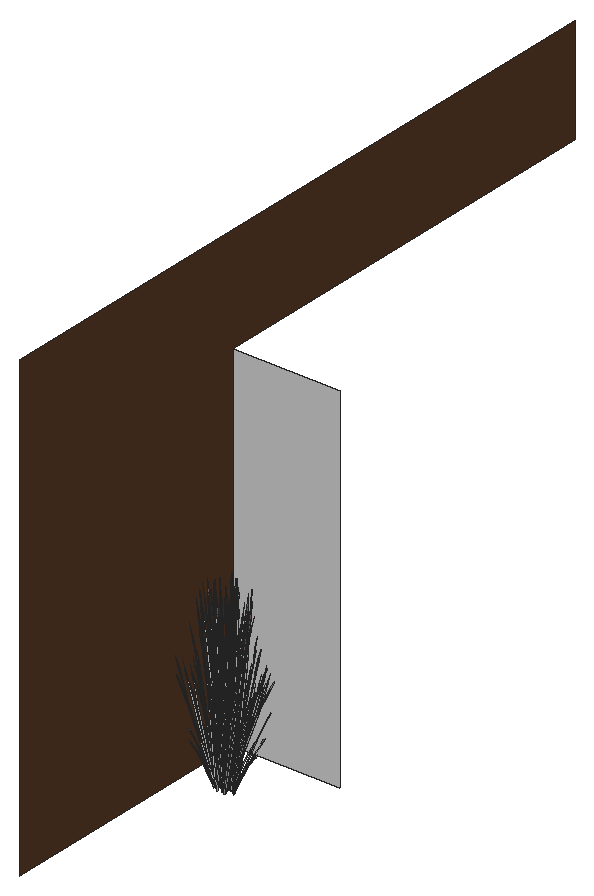
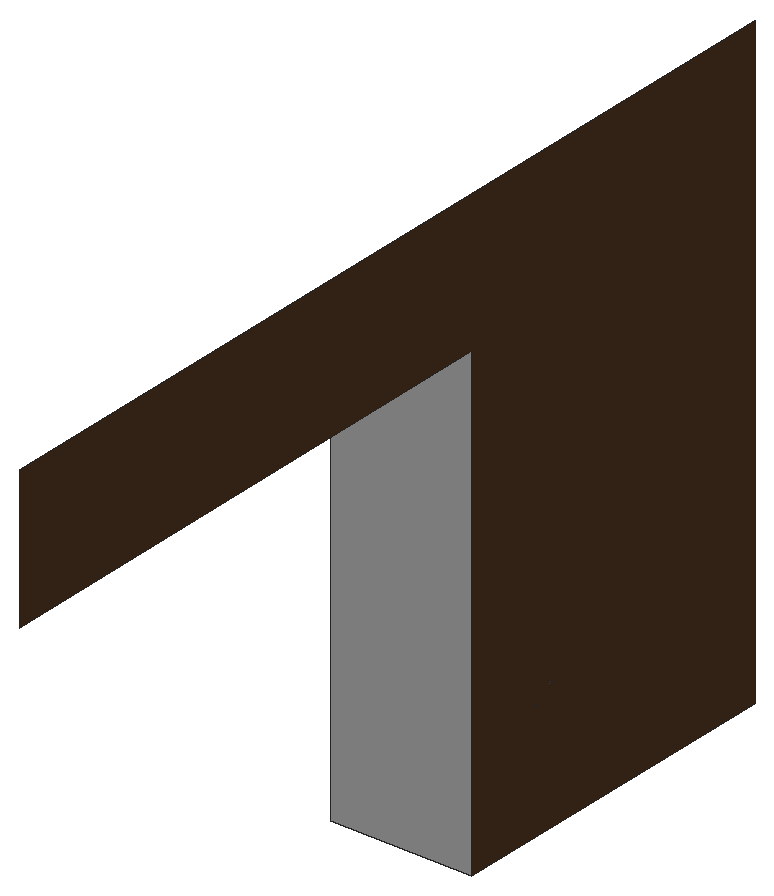
# SketchUp Ruby script. Lengths in inches.
U = 1.inch
M = Sketchup.active_model
def pt(a) = Geom::Point3d.new(a.map { |v| v * U })
def face(e, loops, mat)
  f = e.add_face(loops[0].map { |a| pt(a) })
  loops[1..].each { |l| e.add_face(l.map { |a| pt(a) }).erase! }
  f.material = f.back_material = mat if mat
  f
end
# faces: each face lists its corners as indices into pts; further lists are holes
def faces(e, pts, list, mat = nil) = list.each { |f| face(e, (f[0].is_a?(Array) ? f : [f]).map { |l| l.map { |i| pts[i] } }, mat) }
# xy, xz, yz: faces in a plane at the given z, y or x. An outline is a flat list of corners, or four numbers for a rectangle; further outlines are holes
def ring(l) = l.size == 4 ? [[l[0], l[1]], [l[2], l[1]], [l[2], l[3]], [l[0], l[3]]] : l.each_slice(2).to_a
def flat(e, list, mat, &to3) = list.each { |f| face(e, (f[0].is_a?(Array) ? f : [f]).map { |l| ring(l).map { |u, v| to3.(u, v) } }, mat) }
def xy(e, z, list, mat = nil) = flat(e, list, mat) { |x, y| [x, y, z] }
def xz(e, y, list, mat = nil) = flat(e, list, mat) { |x, z| [x, y, z] }
def yz(e, x, list, mat = nil) = flat(e, list, mat) { |y, z| [x, y, z] }
def lines(e, pts, list) = list.each { |a, b| e.add_line(pt(pts[a]), pt(pts[b])) }
# prism: a flat outline (further loops are holes) pulled along v
def prism(e, loops, v, mat = nil)
  f = face(e, loops, mat); d = Geom::Vector3d.new(v.map { |x| x * U })
  f.pushpull(f.normal.samedirection?(d) ? d.length : -d.length)
end
def box(e, o, s, mat = nil) = prism(e, [[o, [o[0] + s[0], o[1], o[2]], [o[0] + s[0], o[1] + s[1], o[2]], [o[0], o[1] + s[1], o[2]]]], [0, 0, s[2]], mat)
def at(x, y, z, deg = 0) = Geom::Transformation.translation(pt([x, y, z])) * Geom::Transformation.rotation(ORIGIN, Z_AXIS, deg.degrees)
def axes(o, x, y, z) = Geom::Transformation.new([*x, 0, *y, 0, *z, 0, *pt(o).to_a, 1])
def part(name) = M.definitions.add(name)
# library, detail: a bought-in or finely detailed component or shape, given as its bounding box
def library(name, o, s) = part(name).tap { |d| box(d.entities, o, s) }
def detail(e, o, s) = box(e.add_group.entities, o, s)
def put(e, d, t, mat = nil) = e.add_instance(d, t).tap { |i| i.material = mat if mat }
def group(e, t, mat = nil) = e.add_group.tap { |g| g.transformation = t; g.material = mat if mat }.entities
root = M.entities
M.materials.add("LightPink_Translucent").color = [144, 107, 117]
M.materials["LightPink_Translucent"].alpha = 0.75
M.materials.add("Wood_Veneer_15_1K").color = [81, 54, 35]
M.materials.add("[_0053_Ivory_]").color = [200, 200, 200]
c1 = part("blade")
p = [[2.15,0.21,22],[0,0.17,0],[0.09,0.45,0],[2.18,0.31,22],[2.29,0.31,22],[0.38,0.45,0],
  [2.48,0.24,33],[2.49,0.24,33],[2.48,0.22,33]]
faces(c1.entities,p,[[0,1,2,3],[4,5,2,3],[6,3,4,7],[8,0,3,6]])
c2 = part("seeds")
p = [[0.3,-0.1,1.38],[-0.01,-0.03,1.59],[-0.01,-0.03,0.03],[0.14,-0.07,-0.07],[0.29,-0.03,3],[0.15,0.01,3.11]]
faces(c2.entities,p,[[0,1,2,3],[1,0,4,5]],"LightPink_Translucent")
c3 = part("blade with seeds")
put(c3.entities,c1,at(0,0,0))
put(c3.entities,c2,axes([2.4,0.25,30.99],[1.5799,-0.05474,1.17369],[-0.12525,1.92788,0.29478],[-0.07173,-0.02425,1.56792]))
xz(root,359.15,[[617.51,252,653.51,372]],"[_0053_Ivory_]")
yz(root,617.51,[[269.15,252,359.15,252,359.15,372,503.15,372,503.15,408,269.15,408]],"Wood_Veneer_15_1K")
put(root,c3,axes([631.41,334.82,253.68],[0.56663,0.1556,-0.30978],[-0.14267,0.54795,0.30978],[0.11423,-0.06319,1.38974]),"[_0053_Ivory_]")
put(root,c3,axes([629.83,335.5,256.63],[-0.60713,-0.01514,-0.71045],[0.04078,-0.63759,0.08574],[-0.25721,-0.06729,1.00501]),"[_0053_Ivory_]")
put(root,c3,axes([629.8,336.73,253.98],[-0.56493,0.5287,0.30756],[-0.56528,-0.52313,-0.36492],[-0.01973,-0.15014,1.64885]),"[_0053_Ivory_]")
put(root,c3,axes([631.6,336.97,254.09],[0.68433,0.30479,0.24065],[-0.32934,0.63331,0.50002],[0,-0.14599,1.60543]),"[_0053_Ivory_]")
put(root,c3,axes([631.33,337.83,254.09],[0.16098,-0.74515,-0.23429],[0.76326,0.12989,0.51271],[-0.13337,-0.1029,1.5644]),"[_0053_Ivory_]")
put(root,c3,axes([629.63,335.63,256.33],[-0.44101,0.41656,-0.51099],[-0.38623,-0.44004,-0.3958],[-0.22407,-0.06338,0.97773]),"[_0053_Ivory_]")
put(root,c3,axes([628.64,336.18,254.42],[0.38775,-0.045,1.1486],[-0.24596,0.39648,0.84392],[-0.19161,-0.05948,0.25299]),"[_0053_Ivory_]")
put(root,c3,axes([631.38,336.55,254.37],[-0.65953,0.03882,0.44739],[-0.05964,-0.64439,-0.21531],[0.11807,-0.06531,1.43643]),"[_0053_Ivory_]")
put(root,c3,axes([629.68,337.02,254.13],[0,0.62885,0.49651],[-0.67951,0,0],[0,-0.14322,1.57504]),"[_0053_Ivory_]")
put(root,c3,axes([634.45,337.16,256.33],[0.16454,-0.57202,-0.51099],[0.56413,0.19607,-0.3958],[0.22713,-0.05245,0.97773]),"[_0053_Ivory_]")
put(root,c3,axes([633.55,334.83,254.03],[0.37973,-0.63014,0],[0.6353,0.35142,-0.51607],[0.14469,0.08004,1.63711]),"[_0053_Ivory_]")
put(root,c3,axes([629.08,336.07,255.53],[0.25192,-0.01424,1.71376],[-0.16712,0.61729,0.13857],[-0.35901,-0.03818,0.73262]),"[_0053_Ivory_]")
put(root,c3,axes([631.28,337.53,253.86],[-0.36485,-0.52782,-0.44739],[0.55265,-0.37168,0.21531],[-0.11807,-0.06531,1.43643]),"[_0053_Ivory_]")
put(root,c3,axes([631.36,336.78,254.01],[0.26406,0.70318,0.45755],[-0.7545,0.24452,0.17955],[0.00922,-0.12921,1.58856]),"[_0053_Ivory_]")
put(root,c3,axes([635.05,337.32,253.64],[-0.39118,0.07547,1.41583],[-0.06226,-0.6007,0.08104],[0.27398,-0.09092,0.80566]),"[_0053_Ivory_]")
put(root,c3,axes([635.76,336.79,253.91],[-0.37654,-0.40212,-0.06488],[0.4124,-0.36845,-0.29416],[0.11685,-0.02594,0.97024]),"[_0053_Ivory_]")
put(root,c3,axes([631.22,337.33,254.37],[-0.29468,0.56664,0.44739],[-0.61229,-0.27271,-0.21531],[0,-0.13062,1.43643]),"[_0053_Ivory_]")
put(root,c3,axes([632.31,336.84,253.86],[0,-0.72763,0],[0.75945,0,0],[0,0,1.79456]),"[_0053_Ivory_]")
put(root,c3,axes([633.23,335.16,254.13],[-0.56842,-0.31443,0.49651],[0.33976,-0.56381,0],[0.12946,0.07161,1.57504]),"[_0053_Ivory_]")
put(root,c3,axes([634.34,337.37,256.63],[0.53369,-0.27773,-0.71045],[0.29743,0.5717,0.08574],[0.25786,-0.06494,1.00501]),"[_0053_Ivory_]")
put(root,c3,axes([630.95,337.73,253.71],[-0.63179,-0.1031,-0.62353],[0.13332,-0.63596,-0.16365],[-0.18854,-0.07706,1.37633]),"[_0053_Ivory_]")
put(root,c3,axes([631.95,336.38,254.01],[-0.50358,0.57069,0.45755],[-0.59827,-0.50377,0.17955],[0.1214,-0.05695,1.58856]),"[_0053_Ivory_]")
put(root,c3,axes([632.5,337.4,253.95],[-0.56493,-0.54126,-0.06131],[0.56528,-0.54159,0],[-0.01973,-0.0189,1.75571]),"[_0053_Ivory_]")
put(root,c3,axes([631.07,335.44,254.13],[-0.17545,0.62497,0.17642],[-0.64204,-0.17686,0.35086],[0.11091,-0.00304,1.60407]),"[_0053_Ivory_]")
put(root,c3,axes([630.81,335.95,253.25],[-0.59782,0.25177,1.28929],[-0.19028,-0.72239,0.50096],[0.36709,0.01202,1.46642]),"[_0053_Ivory_]")
put(root,c3,axes([632.41,336.14,254.27],[0.11717,-0.56122,0.1448],[0.57245,0.09742,-0.41347],[0.10418,0.05763,1.26744]),"[_0053_Ivory_]")
put(root,c3,axes([631.42,337.47,254.01],[0.76764,0.13249,0.45755],[-0.15622,0.74829,0.17955],[-0.11218,-0.07226,1.58856]),"[_0053_Ivory_]")
put(root,c3,axes([635.48,336.93,253.15],[-0.03174,-0.09547,1.76342],[0.22015,-0.55846,-0.26939],[0.22208,-0.00803,0.30037]),"[_0053_Ivory_]")
put(root,c3,axes([628.92,336.83,253.15],[0.0154,0.09911,1.76342],[-0.31051,0.51756,-0.26939],[-0.22056,-0.02609,0.30037]),"[_0053_Ivory_]")
put(root,c3,axes([632.17,336.28,254.37],[-0.36485,-0.52782,0.44739],[0.55265,-0.37168,-0.21531],[0.11807,0.06531,1.43643]),"[_0053_Ivory_]")
put(root,c3,axes([630.28,338.7,253.68],[-0.14267,-0.54795,-0.30978],[0.56663,-0.1556,0.30978],[-0.11423,-0.06319,1.38974]),"[_0053_Ivory_]")
put(root,c3,axes([631.01,338.66,254.13],[0.65264,-0.16691,0.17642],[0.16115,0.62115,0.35086],[-0.05821,-0.0905,1.60407]),"[_0053_Ivory_]")
put(root,c3,axes([632.35,336.32,254.32],[0.61322,-0.4175,-0.29095],[0.40778,0.58992,-0.50002],[0.1513,0.05991,1.59708]),"[_0053_Ivory_]")
put(root,c3,axes([634.79,337.42,256.18],[0.50475,0.17543,-0.35414],[-0.14722,0.5118,0.4572],[0.20322,-0.04693,0.87481]),"[_0053_Ivory_]")
put(root,c3,axes([630.125,338.93,253.67],[-0.56842,-0.31443,-0.49651],[0.33976,-0.56381,0],[-0.12946,-0.07161,1.57504]),"[_0053_Ivory_]")
put(root,c3,axes([633.9,335.21,253.67],[0.56842,0.31443,-0.49651],[-0.33976,0.56381,0],[0.12946,0.07161,1.57504]),"[_0053_Ivory_]")
put(root,c3,axes([628.86,336.6,256.18],[-0.50475,-0.17543,-0.35414],[0.14722,-0.5118,0.4572],[-0.20322,0.04693,0.87481]),"[_0053_Ivory_]")
put(root,c3,axes([632.82,337,253.86],[0.67951,0,0],[0,0.65103,0],[0,0,1.78407]),"[_0053_Ivory_]")
put(root,c3,axes([631.67,337.82,254.32],[-0.61322,0.4175,-0.29095],[-0.40778,-0.58992,-0.50002],[-0.1513,-0.05991,1.59708]),"[_0053_Ivory_]")
put(root,c3,axes([633.01,335.48,254.13],[-0.65264,0.16691,0.17642],[-0.16115,-0.62115,0.35086],[0.05821,0.0905,1.60407]),"[_0053_Ivory_]")
put(root,c3,axes([633.42,336.79,255.53],[-0.25192,0.01424,1.71376],[0.16712,-0.61729,0.13857],[0.35901,0.03818,0.73262]),"[_0053_Ivory_]")
put(root,c3,axes([633.74,335.44,253.68],[0.14267,0.54795,-0.30978],[-0.56663,0.1556,0.30978],[0.11423,0.06319,1.38974]),"[_0053_Ivory_]")
put(root,c3,axes([632.6,336.67,254.03],[-0.76764,-0.13249,0.49198],[0.15622,-0.74829,0.19306],[0.11218,0.07226,1.70813]),"[_0053_Ivory_]")
put(root,c3,axes([631.99,338.52,253.86],[-0.19817,-0.54216,0],[0.56587,-0.18986,0],[0,0,1.54371]),"[_0053_Ivory_]")
put(root,c3,axes([631.61,338,254.27],[-0.11717,0.56122,0.1448],[-0.57245,-0.09742,-0.41347],[-0.10418,-0.05763,1.26744]),"[_0053_Ivory_]")
put(root,c3,axes([632.73,338.44,253.84],[0.63764,-0.21337,-0.19198],[0.22406,0.61462,0.00008],[0.07038,-0.02358,1.73897]),"[_0053_Ivory_]")
put(root,c3,axes([632.95,338.7,254.13],[0.17545,-0.62497,0.17642],[0.64204,0.17686,0.35086],[-0.11091,0.00304,1.60407]),"[_0053_Ivory_]")
put(root,c3,axes([632.81,337.28,253.87],[0.42396,0.40619,0],[-0.42396,0.40619,0],[0,0,1.69266]),"[_0053_Ivory_]")
put(root,c3,axes([630.4,336.52,255],[0.17264,-0.09097,1.77064],[0.05953,0.63516,0.13857],[-0.37394,0.08428,0.63284]),"[_0053_Ivory_]")
put(root,c3,axes([633.95,337.1,254.13],[-0.47719,-0.45806,0.17642],[0.48088,-0.44429,0.35086],[-0.0527,0.09355,1.60407]),"[_0053_Ivory_]")
put(root,c3,axes([633.07,336.41,253.71],[0.63179,0.1031,-0.62353],[-0.13332,0.63596,-0.16365],[0.18854,0.07706,1.37633]),"[_0053_Ivory_]")
put(root,c3,axes([635.86,337.52,254.42],[-0.37526,0.10382,1.1486],[0.17664,-0.42906,0.84392],[0.19907,0.02936,0.25299]),"[_0053_Ivory_]")
put(root,c3,axes([631.85,338.76,253.85],[-0.61229,-0.28233,0],[0.29468,-0.58663,0],[0,0,1.62707]),"[_0053_Ivory_]")
put(root,c3,axes([632.36,338.01,254.12],[-0.59306,-0.50614,-0.25192],[0.49904,-0.56836,0.5513],[-0.1597,0.05921,1.68216]),"[_0053_Ivory_]")
put(root,c3,axes([630.8,338.98,254.13],[0.56842,0.31443,0.49651],[-0.33976,0.56381,0],[-0.12946,-0.07161,1.57504]),"[_0053_Ivory_]")
put(root,c3,axes([632.8,336.81,254.37],[0.29468,-0.56664,0.44739],[0.61229,0.27271,-0.21531],[0,0.13062,1.43643]),"[_0053_Ivory_]")
put(root,c3,axes([632.6875,337.13,253.95],[0,0.72727,-0.05637],[-0.75945,0,0],[0,0.02286,1.79368]),"[_0053_Ivory_]")
put(root,c3,axes([629.21,336.86,256.33],[-0.16454,0.57202,-0.51099],[-0.56413,-0.19607,-0.3958],[-0.22713,0.05245,0.97773]),"[_0053_Ivory_]")
put(root,c3,axes([632.74,336.61,253.86],[0.36485,0.52782,-0.44739],[-0.55265,0.37168,0.21531],[0.11807,0.06531,1.43643]),"[_0053_Ivory_]")
put(root,c3,axes([635.21,338.85,255.58],[-0.11624,-0.52862,-0.03492],[0.54943,-0.12153,-0.15832],[0.11473,0.03351,0.52218]),"[_0053_Ivory_]")
put(root,c3,axes([630.47,339.3125,254.03],[-0.37973,0.63014,0],[-0.6353,-0.35142,-0.51607],[-0.14469,-0.08004,1.63711]),"[_0053_Ivory_]")
put(root,c3,axes([634.35,337.12,254.13],[0,-0.62885,0.49651],[0.67951,0,0],[0,0.14322,1.57504]),"[_0053_Ivory_]")
put(root,c3,axes([632.65,337.59,254.37],[0.65953,-0.03882,0.44739],[0.05964,0.64439,-0.21531],[-0.11807,0.06531,1.43643]),"[_0053_Ivory_]")
put(root,c3,axes([633.06,336.9375,254.27],[0.56587,-0.18339,0.1448],[0.19817,0.52368,-0.41347],[0,0.11525,1.26744]),"[_0053_Ivory_]")
put(root,c3,axes([632.06,337.9,253.86],[-0.65953,0.03882,-0.44739],[-0.05964,-0.64439,0.21531],[-0.11807,0.06531,1.43643]),"[_0053_Ivory_]")
put(root,c3,axes([635.16,338.21,254.24],[-0.14627,-0.15466,1.43002],[0.19032,-0.51164,-0.30754],[0.29594,0.06931,0.61141]),"[_0053_Ivory_]")
put(root,c3,axes([632.55,338.77,253.86],[0.61229,0.28233,0],[-0.29468,0.58663,0],[0,0,1.74954]),"[_0053_Ivory_]")
put(root,c3,axes([632.79,339.4,253.85],[-0.37499,-0.63235,-0.05142],[0.6353,-0.35142,0.51607],[-0.15655,0.0602,1.6363]),"[_0053_Ivory_]")
put(root,c3,axes([632.66,337.87,254.27],[0.44871,0.37783,0.1448],[-0.37428,0.42627,-0.41347],[-0.10418,0.05763,1.26744]),"[_0053_Ivory_]")
put(root,c3,axes([629.1875,337.16,255.53],[0.21074,-0.13302,1.71376],[0.17741,0.61464,0.13857],[-0.33083,0.13891,0.73262]),"[_0053_Ivory_]")
put(root,c3,axes([633.82,338.52,256.63],[0.60713,0.01514,-0.71045],[-0.04078,0.63759,0.08574],[0.25721,0.06729,1.00501]),"[_0053_Ivory_]")
put(root,c3,axes([633.13,339.03,254.13],[0.56842,-0.31443,0.49651],[0.33976,0.56381,0],[-0.12946,0.07161,1.57504]),"[_0053_Ivory_]")
put(root,c3,axes([632.32,338.54,253.94],[0.26406,0.72244,-0.06012],[-0.7545,0.25315,0],[0.00922,0.02523,1.72173]),"[_0053_Ivory_]")
put(root,c3,axes([632.62,339.32,253.68],[-0.56663,-0.1556,-0.30978],[0.14267,-0.54795,0.30978],[-0.11423,0.06319,1.38974]),"[_0053_Ivory_]")
put(root,c3,axes([628.53,338.21,254.24],[0.21107,0.05162,1.43002],[0.13604,0.52729,-0.30754],[-0.28671,0.0987,0.61141]),"[_0053_Ivory_]")
put(root,c3,axes([634.81,337.23,254.03],[0.75945,0,0],[0,0.70283,-0.51607],[0,0.16007,1.63711]),"[_0053_Ivory_]")
put(root,c3,axes([634.51,337.59,253.85],[-0.75908,-0.00503,-0.04976],[0,-0.70283,0.49943],[-0.02386,0.16,1.58352]),"[_0053_Ivory_]")
put(root,c3,axes([632.86,336.98,254.32],[0.68399,0.30005,-0.29095],[-0.32934,0.63331,-0.50002],[0.0215,0.15549,1.59708]),"[_0053_Ivory_]")
put(root,c3,axes([628.09,339.3125,254.42],[0.25312,-0.28501,1.1486],[0.09988,0.45119,0.84392],[-0.18292,0.08079,0.25299]),"[_0053_Ivory_]")
put(root,c3,axes([634.18,338.79,256.18],[0.34557,0.39372,-0.35414],[-0.39459,0.37271,0.4572],[0.20048,0.05671,0.87481]),"[_0053_Ivory_]")
put(root,c3,axes([634.35,337.69,253.68],[-0.42396,0.39235,-0.30978],[-0.42396,-0.39235,0.30978],[0,0.12637,1.38974]),"[_0053_Ivory_]")
put(root,c3,axes([632.52,337.73,254.32],[0.07077,0.71755,-0.29095],[-0.73712,0.04339,-0.50002],[-0.1298,0.09558,1.59708]),"[_0053_Ivory_]")
put(root,c3,axes([632.79,337.45,253.86],[-0.29468,0.56664,-0.44739],[-0.61229,-0.27271,0.21531],[0,0.13062,1.43643]),"[_0053_Ivory_]")
put(root,c3,axes([629.04,338.08,256.18],[-0.52868,0.08987,-0.35414],[-0.1396,-0.51376,0.4572],[-0.1515,0.13799,0.87481]),"[_0053_Ivory_]")
put(root,c3,axes([632.08,338.28,253.71],[-0.40909,0.47266,-0.62353],[-0.50819,-0.4286,-0.16365],[-0.16393,0.11791,1.37633]),"[_0053_Ivory_]")
put(root,c3,axes([632.81,339.07,253.98],[0.76036,0.2044,0.30756],[-0.19023,0.7306,-0.36492],[-0.12585,0.09144,1.64885]),"[_0053_Ivory_]")
put(root,c3,axes([632.75,339.57,253.67],[-0.56842,0.31443,-0.49651],[-0.33976,-0.56381,0],[-0.12946,0.07161,1.57504]),"[_0053_Ivory_]")
put(root,c3,axes([634.64,337.71,253.67],[0,0.62885,-0.49651],[-0.67951,0,0],[0,0.14322,1.57504]),"[_0053_Ivory_]")
put(root,c3,axes([632.94,337.78,255.53],[-0.2256,-0.10835,1.71376],[0.46687,-0.45453,0.13857],[0.29098,0.20505,0.73262]),"[_0053_Ivory_]")
put(root,c3,axes([633.78,339.01,254.42],[-0.34197,-0.18082,1.1486],[0.44156,-0.18372,0.84392],[0.1191,0.15563,0.25299]),"[_0053_Ivory_]")
put(root,c3,axes([629.96,337.57,255.53],[0.1517,-0.19322,1.71376],[0.38303,0.52154,0.13857],[-0.26271,0.23751,0.73262]),"[_0053_Ivory_]")
put(root,c3,axes([629.48,338.14,256.33],[0.15602,0.5742,-0.51099],[-0.59087,0.10045,-0.3958],[-0.16933,0.15423,0.97773]),"[_0053_Ivory_]")
put(root,c3,axes([633.27,339.47,254.03],[0.37973,0.63014,0],[-0.6353,0.35142,-0.51607],[-0.14469,0.08004,1.63711]),"[_0053_Ivory_]")
put(root,c3,axes([633.87,339.68,253.15],[0.04425,-0.09079,1.76342],[0.55709,-0.26738,-0.26939],[0.16889,0.13839,0.30037]),"[_0053_Ivory_]")
put(root,c3,axes([632.94,336.98,254.5],[-0.01659,-0.59209,1.41272],[0.75089,0.15348,0.59816],[-0.1776,0.32398,1.3335]),"[_0053_Ivory_]")
put(root,c3,axes([633.14,337.62,253.75],[0.2227,0.57576,-0.69212],[-0.64151,0.20736,-0.18165],[0.02462,0.19497,1.52773]),"[_0053_Ivory_]")
put(root,c3,axes([628.76,339.6,253.15],[0.08147,0.06283,1.76342],[0.13814,0.58211,-0.26939],[-0.18056,0.12413,0.30037]),"[_0053_Ivory_]")
put(root,c3,axes([633,339.26,256.33],[0.59932,-0.14948,-0.51099],[0.10484,0.56611,-0.3958],[0.16097,0.16223,0.97773]),"[_0053_Ivory_]")
put(root,c3,axes([633.83,339.83,254.32],[-0.38947,-0.01972,1.0506],[0.25721,-0.41888,0.58006],[0.15386,0.14882,0.8241]),"[_0053_Ivory_]")
put(root,c3,axes([629.84,338.05,255.53],[0.11309,-0.21615,1.71376],[0.47441,0.44731,0.13857],[-0.21402,0.27879,0.73262]),"[_0053_Ivory_]")
put(root,c3,axes([632.56,338.82,254.24],[0.01072,-0.20846,1.43002],[0.51218,-0.23285,-0.30754],[0.15811,0.2495,0.61141]),"[_0053_Ivory_]")
put(root,c3,axes([629.97,339.27,256.18],[-0.41095,0.33109,-0.35414],[-0.38901,-0.37805,0.4572],[-0.05919,0.19208,0.87481]),"[_0053_Ivory_]")
put(root,c3,axes([630.24,340.56,254.42],[-0.01572,-0.37392,1.1486],[0.39276,0.26669,0.84392],[-0.07724,0.17822,0.25299]),"[_0053_Ivory_]")
put(root,c3,axes([631.27,339.66,253.15],[0.09829,-0.03422,1.76342],[0.59126,0.18834,-0.26939],[0.01729,0.21228,0.30037]),"[_0053_Ivory_]")
put(root,c3,axes([630.38,339.11,256.66],[0.43478,0.42253,-0.5672],[-0.45929,0.37004,-0.43934],[-0.06615,0.21468,1.08528]),"[_0053_Ivory_]")
put(root,c3,axes([629.91,339.75,254.48],[0.55175,-0.11136,0.06507],[0.12684,0.44864,-0.86304],[-0.03498,0.22711,0.7736]),"[_0053_Ivory_]")
put(root,c3,axes([631.67,339.52,256.33],[0.59704,0.15764,-0.51099],[-0.20464,0.54049,-0.3958],[0.05475,0.21761,0.97773]),"[_0053_Ivory_]")
put(root,c3,axes([632.01,338.41,255.53],[-0.13883,-0.2019,1.71376],[0.64153,-0.16998,0.13857],[0.14499,0.31697,0.73262]),"[_0053_Ivory_]")
put(root,c3,axes([631.4,339.85,256.18],[-0.1831,0.48359,-0.35414],[-0.53419,-0.14105,0.4572],[0.04898,0.1947,0.87481]),"[_0053_Ivory_]")
put(root,c3,axes([630.25,338.92,256.99],[-0.0158,0.58168,-0.7886],[-0.66548,-0.03907,0.09517],[-0.07023,0.24643,1.11556]),"[_0053_Ivory_]")
put(root,c3,axes([630.88,338.51,255.53],[-0.01487,-0.24136,1.71376],[0.64429,0.16012,0.13857],[-0.03985,0.34396,0.73262]),"[_0053_Ivory_]")
put(root,c3,axes([631.46,339.42,256.63],[0.28988,0.51132,-0.71045],[-0.59671,0.28496,0.08574],[0.06778,0.24706,1.00501]),"[_0053_Ivory_]")
put(root,c3,axes([629.78,340.22,254.24],[0.19166,-0.0992,1.43002],[0.4732,0.29912,-0.30754],[-0.14084,0.25882,0.61141]),"[_0053_Ivory_]")
put(root,c3,axes([630.03,339.74,255.02],[0.01334,-0.32463,1.54345],[0.60018,0.17147,0.21329],[-0.052,0.34598,0.72882]),"[_0053_Ivory_]")
